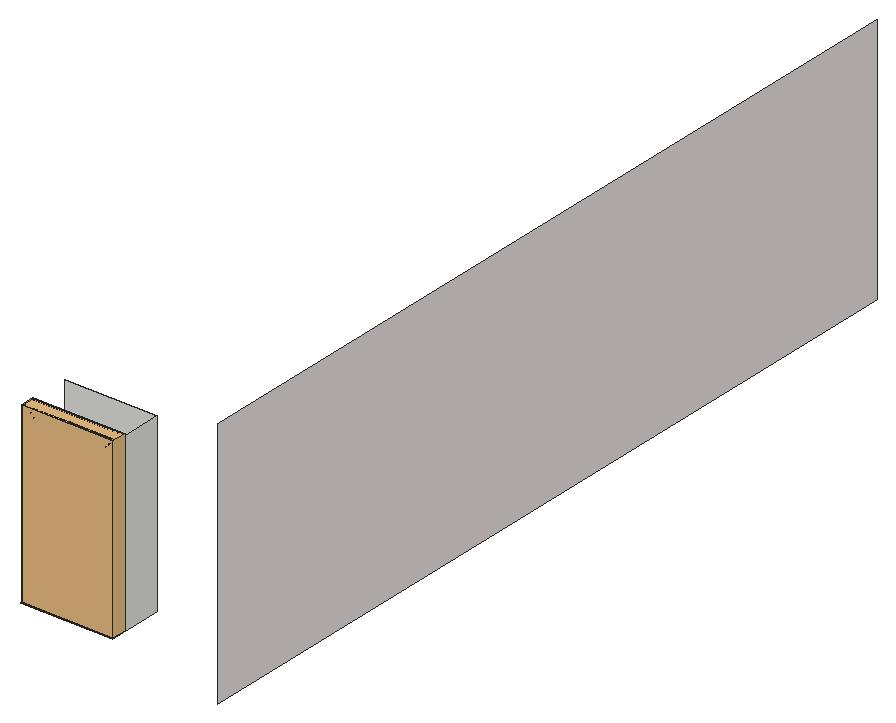
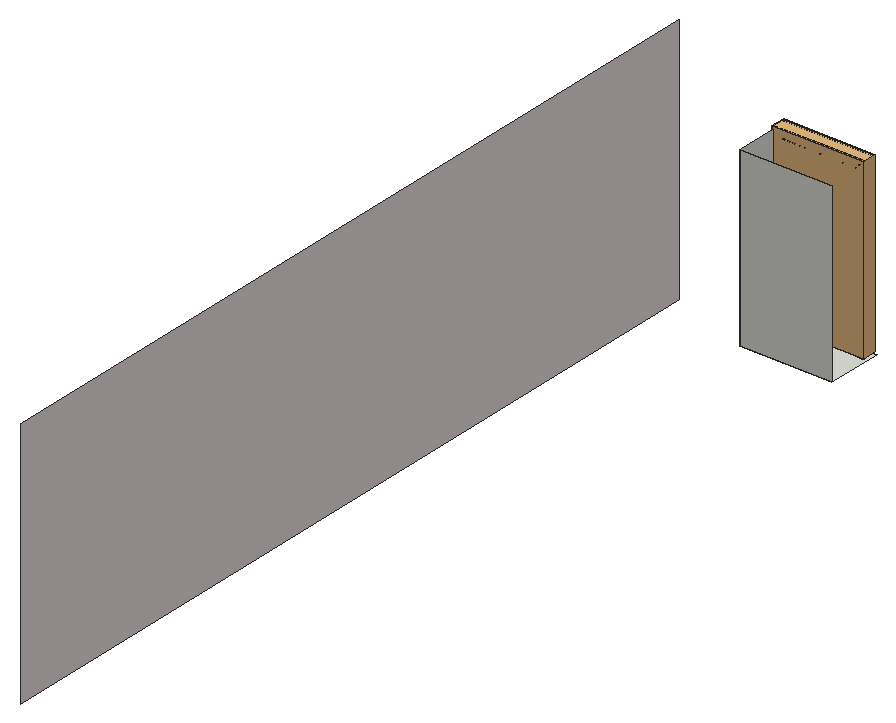
# SketchUp Ruby script. Lengths in inches.
U = 1.inch
M = Sketchup.active_model
def pt(a) = Geom::Point3d.new(a.map { |v| v * U })
def face(e, loops, mat)
  f = e.add_face(loops[0].map { |a| pt(a) })
  loops[1..].each { |l| e.add_face(l.map { |a| pt(a) }).erase! }
  f.material = f.back_material = mat if mat
  f
end
# faces: each face lists its corners as indices into pts; further lists are holes
def faces(e, pts, list, mat = nil) = list.each { |f| face(e, (f[0].is_a?(Array) ? f : [f]).map { |l| l.map { |i| pts[i] } }, mat) }
# xy, xz, yz: faces in a plane at the given z, y or x. An outline is a flat list of corners, or four numbers for a rectangle; further outlines are holes
def ring(l) = l.size == 4 ? [[l[0], l[1]], [l[2], l[1]], [l[2], l[3]], [l[0], l[3]]] : l.each_slice(2).to_a
def flat(e, list, mat, &to3) = list.each { |f| face(e, (f[0].is_a?(Array) ? f : [f]).map { |l| ring(l).map { |u, v| to3.(u, v) } }, mat) }
def xy(e, z, list, mat = nil) = flat(e, list, mat) { |x, y| [x, y, z] }
def xz(e, y, list, mat = nil) = flat(e, list, mat) { |x, z| [x, y, z] }
def yz(e, x, list, mat = nil) = flat(e, list, mat) { |y, z| [x, y, z] }
def lines(e, pts, list) = list.each { |a, b| e.add_line(pt(pts[a]), pt(pts[b])) }
# prism: a flat outline (further loops are holes) pulled along v
def prism(e, loops, v, mat = nil)
  f = face(e, loops, mat); d = Geom::Vector3d.new(v.map { |x| x * U })
  f.pushpull(f.normal.samedirection?(d) ? d.length : -d.length)
end
def box(e, o, s, mat = nil) = prism(e, [[o, [o[0] + s[0], o[1], o[2]], [o[0] + s[0], o[1] + s[1], o[2]], [o[0], o[1] + s[1], o[2]]]], [0, 0, s[2]], mat)
def at(x, y, z, deg = 0) = Geom::Transformation.translation(pt([x, y, z])) * Geom::Transformation.rotation(ORIGIN, Z_AXIS, deg.degrees)
def axes(o, x, y, z) = Geom::Transformation.new([*x, 0, *y, 0, *z, 0, *pt(o).to_a, 1])
def part(name) = M.definitions.add(name)
# library, detail: a bought-in or finely detailed component or shape, given as its bounding box
def library(name, o, s) = part(name).tap { |d| box(d.entities, o, s) }
def detail(e, o, s) = box(e.add_group.entities, o, s)
def put(e, d, t, mat = nil) = e.add_instance(d, t).tap { |i| i.material = mat if mat }
def group(e, t, mat = nil) = e.add_group.tap { |g| g.transformation = t; g.material = mat if mat }.entities
root = M.entities
M.materials.add("Generic\#5").color = [232, 222, 222]
M.materials.add("Material \#0").color = [86, 53, 35]
M.materials.add("Material \#1").color = [140, 140, 140]
c1 = part("3DGeom~19_Defintion")
xy(c1.entities,0,[[-6.28,-215.79,-994.45,-208.55,-13.52,-208.55],[-994.45,-215.79,-994.45,-208.55,-6.28,-215.79],[-6.28,-215.79,-13.52,-208.55,-13.52,0],[-6.28,-215.79,-13.52,0,-6.28,0],[-13.52,0,-13.52,208.55,-6.28,215.79],
  [-13.52,0,-6.28,215.79,-6.28,0],[-994.45,208.55,-6.28,215.79,-13.52,208.55],[-994.45,208.55,-994.45,215.79,-6.28,215.79]],"Material \#0")
p = [[-13.52,-208.55,0],[-994.45,-208.55,0],[-994.45,-207.81,0.07],[-14.25,-207.81,0.07],[-13.52,-208.55,0],[-14.25,-207.81,0.07],
  [-14.25,0,0.07],[-13.52,0,0],[-13.52,208.55,0],[-14.25,207.81,0.07],[-13.52,208.55,0],[-14.25,207.81,0.07],
  [-994.45,207.81,0.07],[-994.45,208.55,0],[-994.45,-207.21,0.27],[-994.45,-207.21,0.27],[-14.86,-207.21,0.27],[-14.86,-207.21,0.27],
  [-14.86,0,0.27],[-14.86,0,0.27],[-14.86,0,0.27],[-14.86,0,0.27],[-14.86,207.21,0.27],[-14.86,207.21,0.27],
  [-994.45,207.21,0.27],[-994.45,207.21,0.27],[-14.86,-207.21,0.27],[-994.45,-207.21,0.27],[-994.45,-206.74,0.6],[-15.33,-206.74,0.6],
  [-14.86,-207.21,0.27],[-15.33,-206.74,0.6],[-15.33,0,0.6],[-14.86,0,0.27],[-14.86,207.21,0.27],[-15.33,206.74,0.6],
  [-14.86,207.21,0.27],[-15.33,206.74,0.6],[-994.45,206.74,0.6],[-994.45,207.21,0.27],[-994.45,-206.4,1.07],[-15.66,-206.4,1.07],
  [-15.66,-206.4,1.07],[-15.66,0,1.07],[-15.66,206.4,1.07],[-15.66,206.4,1.07],[-994.45,206.4,1.07],[-994.45,-206.2,1.68],
  [-15.86,-206.2,1.68],[-15.86,-206.2,1.68],[-15.86,0,1.68],[-15.86,206.2,1.68],[-15.86,206.2,1.68],[-994.45,206.2,1.68],
  [-994.45,-206.13,2.41],[-15.93,-206.13,2.41],[-15.93,-206.13,2.41],[-15.93,0,2.41],[-15.93,206.13,2.41],[-15.93,206.13,2.41],
  [-994.45,206.13,2.41],[-994.45,-206.13,71.16],[-994.45,-206.22,71.59],[-15.79,-206.28,71.53],[-15.79,-206.28,71.53],[-15.84,0,71.59],
  [-15.93,0,71.16],[-15.79,206.28,71.53],[-15.79,206.28,71.53],[-994.45,206.22,71.59],[-994.45,206.13,71.16],[-15.79,-206.28,71.53],
  [-994.45,-206.48,71.84],[-994.45,-206.9,71.93],[-15.16,-206.9,71.93],[-15.79,-206.28,71.53],[-15.79,-206.28,71.53],[-15.16,-206.9,71.93],
  [-15.16,0,71.93],[-994.45,-206.48,71.84],[-15.59,0,71.84],[-15.79,-206.28,71.53],[-15.59,0,71.84],[-15.79,206.28,71.53],
  [-15.16,206.9,71.93],[-15.59,0,71.84],[-15.79,206.28,71.53],[-994.45,206.48,71.84],[-15.79,206.28,71.53],[-15.16,206.9,71.93],
  [-994.45,206.9,71.93],[-994.45,206.48,71.84],[-15.79,206.28,71.53],[-994.45,-227.27,72.01],[5.41,-227.47,72.33],[4.78,-226.84,71.93],
  [4.78,-226.84,71.93],[5.41,-227.47,72.33],[5.21,0,72.01],[-994.45,-226.84,71.93],[-994.45,-227.27,72.01],[5.21,0,72.01],
  [4.78,0,71.93],[4.78,226.84,71.93],[5.21,0,72.01],[5.21,0,72.01],[5.41,227.47,72.33],[4.78,226.84,71.93],
  [5.41,227.47,72.33],[-994.45,227.27,72.01],[-994.45,227.27,72.01],[-994.45,226.84,71.93],[-994.45,-227.27,72.01],[-994.45,-227.53,72.27],
  [5.41,-227.47,72.33],[5.41,-227.47,72.33],[5.47,0,72.27],[5.21,0,72.01],[5.41,227.47,72.33],[5.41,227.47,72.33],
  [-994.45,227.53,72.27],[-994.45,227.27,72.01],[-994.45,-227.61,72.7],[-994.45,-227.61,74.4375],[-994.45,-227.61,74.4375],[5.55,-227.61,74.4375],
  [5.55,-227.61,74.4375],[5.55,0,74.4375],[5.55,0,72.7],[5.55,227.61,74.4375],[5.55,227.61,74.4375],[-994.45,227.61,74.4375],
  [-994.45,227.61,74.4375],[-994.45,227.61,72.7]]
faces(c1.entities,p,[[0,1,2],[2,3,0],[4,5,6],[6,7,4],[8,7,6],[6,9,8],[10,11,12],[12,13,10],
  [3,2,14],[15,16,3],[5,17,18],[19,6,5],[9,6,20],[21,22,9],[11,23,24],[25,12,11],
  [26,27,28],[28,29,26],[30,31,32],[32,33,30],[34,33,32],[32,35,34],[36,37,38],[38,39,36],
  [29,28,40],[40,41,29],[31,42,43],[43,32,31],[35,32,43],[43,44,35],[37,45,46],[46,38,37],
  [41,40,47],[47,48,41],[42,49,50],[50,43,42],[44,43,50],[50,51,44],[45,52,53],[53,46,45],
  [48,47,54],[54,55,48],[49,56,57],[57,50,49],[51,50,57],[57,58,51],[52,59,60],[60,53,52],
  [61,62,63],[64,65,66],[66,65,67],[68,69,70],[71,72,73],[73,74,75],[76,77,78],[62,79,63],
  [78,80,76],[81,82,65],[83,80,78],[78,84,83],[65,85,86],[68,87,69],[88,89,90],[90,91,92],
  [93,94,95],[96,97,98],[95,99,100],[101,102,96],[103,102,104],[105,106,103],[107,108,109],[110,111,107],
  [112,113,114],[115,116,117],[117,116,118],[119,120,121],[114,122,123],[124,125,114],[113,122,114],[115,126,127],
  [127,128,115],[115,128,116],[118,128,127],[127,129,118],[116,128,118],[119,130,131],[132,133,119],[119,133,120]],"Material \#0")
c2 = part("3DGeom~15_Defintion")
xy(c2.entities,0,[[-961.58,-251.9,-958.5,-248.8125,-961.58,-237.8],[-961.58,-251.9,28.8,-248.8125,-958.5,-248.8125],[-961.58,-251.9,36.25,-251.9,28.8,-248.8125],[36.25,-251.9,19.98,-239.99,28.8,-248.8125],[36.25,-251.9,22.16,-237.8,19.98,-239.99],
  [-958.5,-248.8125,-958.5,-237.8,-961.58,-237.8],[19.98,-239.99,22.16,-237.8,3.36,-223.37],[-958.5,-237.8,-958.5,-223.37,-961.58,-220.28],[-961.58,-237.8,-958.5,-237.8,-961.58,-220.28],[22.16,-237.8,4.64,-220.28,3.36,-223.37],
  [-958.5,-223.37,4.64,-220.28,-961.58,-220.28],[-958.5,-223.37,3.36,-223.37,4.64,-220.28],[5.29,-219.63,8.375,-218.35,5.29,0],[8.375,-218.35,8.375,0,5.29,0],[5.29,0,8.375,0,5.29,219.63],
  [8.375,0,8.375,218.35,5.29,219.63],[8.375,218.35,22.8125,237.15,5.29,219.63],[-961.58,220.28,-958.5,223.37,-961.58,237.8],[-961.58,220.28,3.36,223.37,-958.5,223.37],[-961.58,220.28,4.64,220.28,3.36,223.37],
  [4.64,220.28,19.98,239.99,3.36,223.37],[4.64,220.28,22.16,237.8,19.98,239.99],[-958.5,223.37,-958.5,237.8,-961.58,237.8],[-958.5,237.8,-958.5,248.8125,-961.58,251.9],[-961.58,237.8,-958.5,237.8,-961.58,251.9],
  [22.16,237.8,28.8,248.8125,19.98,239.99],[22.16,237.8,36.25,251.9,28.8,248.8125],[-958.5,248.8125,36.25,251.9,-961.58,251.9],[-958.5,248.8125,28.8,248.8125,36.25,251.9]],"Material \#0")
xy(c2.entities,7.48,[[-962.79,-238.36,23.37,-238.36,-962.79,-219.67],[23.37,-238.36,4.67,-219.67,-962.79,-219.67],[23.37,-238.36,23.37,0,4.67,-219.67],[4.67,-219.67,23.37,0,4.67,0],[23.37,0,23.37,238.36,4.67,219.67],
  [4.67,0,23.37,0,4.67,219.67],[-962.79,219.67,23.37,238.36,-962.79,238.36],[-962.79,219.67,4.67,219.67,23.37,238.36]],"Material \#0")
xy(c2.entities,63.5625,[[-962.79,-238.36,-962.79,-219.67,4.67,-219.67],[-962.79,-238.36,4.67,-219.67,23.37,-238.36],[23.37,-238.36,4.67,-219.67,23.37,0],[4.67,-219.67,4.67,0,23.37,0],[23.37,0,4.67,219.67,23.37,238.36],
  [4.67,0,4.67,219.67,23.37,0],[-962.79,219.67,-962.79,238.36,4.67,219.67],[4.67,219.67,-962.79,238.36,23.37,238.36]],"Material \#0")
xy(c2.entities,69.64,[[-962.79,-219.62,4.63,-219.62,-962.79,-200.32],[4.63,-219.62,-14.68,-200.32,-962.79,-200.32],[4.63,-219.62,4.63,0,-14.68,-200.32],[-14.68,-200.32,4.63,0,-14.68,0],[-14.68,0,4.63,0,-14.68,200.32],
  [4.63,0,4.63,219.62,-14.68,200.32],[-962.79,200.32,-14.68,200.32,4.63,219.62],[-962.79,200.32,4.63,219.62,-962.79,219.62]],"Material \#0")
xy(c2.entities,71.04,[[-961.58,-251.9,-958.5,-248.8125,28.8,-248.8125],[-961.58,-251.9,-961.58,-237.8,-958.5,-248.8125],[-961.58,-251.9,28.8,-248.8125,36.25,-251.9],[36.25,-251.9,19.98,-239.99,22.16,-237.8],[36.25,-251.9,28.8,-248.8125,19.98,-239.99],
  [-958.5,-248.8125,-961.58,-237.8,-958.5,-237.8],[19.98,-239.99,3.36,-223.37,22.16,-237.8],[-958.5,-237.8,-961.58,-220.28,-958.5,-223.37],[-961.58,-237.8,-961.58,-220.28,-958.5,-237.8],[22.16,-237.8,3.36,-223.37,4.64,-220.28],
  [-958.5,-223.37,-961.58,-220.28,4.64,-220.28],[-958.5,-223.37,4.64,-220.28,3.36,-223.37],[5.29,-219.63,5.29,0,8.375,-218.35],[8.375,-218.35,5.29,0,8.375,0],[5.29,0,5.29,219.63,8.375,0],
  [8.375,0,5.29,219.63,8.375,218.35],[8.375,218.35,5.29,219.63,22.8125,237.15],[-961.58,220.28,-958.5,223.37,3.36,223.37],[-961.58,220.28,-961.58,237.8,-958.5,223.37],[-961.58,220.28,3.36,223.37,4.64,220.28],
  [4.64,220.28,3.36,223.37,19.98,239.99],[4.64,220.28,19.98,239.99,22.16,237.8],[-958.5,223.37,-961.58,237.8,-958.5,237.8],[-958.5,237.8,-961.58,251.9,-958.5,248.8125],[-961.58,237.8,-961.58,251.9,-958.5,237.8],
  [22.16,237.8,19.98,239.99,28.8,248.8125],[22.16,237.8,28.8,248.8125,36.25,251.9],[-958.5,248.8125,-961.58,251.9,36.25,251.9],[-958.5,248.8125,36.25,251.9,28.8,248.8125]],"Material \#0")
xz(c2.entities,-238.36,[[-962.79,63.5625,23.37,63.5625,23.37,72.07],[-962.79,63.5625,23.37,72.07,-962.79,72.07]],"Material \#0")
xz(c2.entities,-219.67,[[-962.79,7.48,4.67,7.48,-962.79,63.5625],[4.67,7.48,4.67,63.5625,-962.79,63.5625]],"Material \#0")
xz(c2.entities,219.67,[[-962.79,7.48,-962.79,63.5625,4.67,7.48],[4.67,7.48,-962.79,63.5625,4.67,63.5625]],"Material \#0")
xz(c2.entities,238.36,[[-962.79,63.5625,-962.79,72.07,23.37,72.07],[-962.79,63.5625,23.37,72.07,23.37,63.5625]],"Material \#0")
yz(c2.entities,4.67,[[-219.67,7.48,0,7.48,-219.67,63.5625],[0,7.48,0,63.5625,-219.67,63.5625],[0,7.48,219.67,63.5625,0,63.5625],[0,7.48,219.67,7.48,219.67,63.5625]],"Material \#0")
yz(c2.entities,23.37,[[-238.36,63.5625,0,63.5625,-238.36,72.07],[0,63.5625,0,72.07,-238.36,72.07],[0,63.5625,238.36,63.5625,238.36,72.07],[0,63.5625,238.36,72.07,0,72.07]],"Material \#0")
p = [[36.9,-251.24,0],[37.21,0,-0.16],[34.125,0,-0.14],[36.9,251.24,0],[33.83,243.81,0.02],[33.83,-243.8,0.02],
  [22.8125,-237.15,0],[24.99,-234.97,-0.01],[5.375,-220.37,0],[23.37,-238.36,7.48],[4.67,-219.67,7.48],[4.67,-219.67,7.48],
  [23.37,-238.36,7.48],[23.37,-238.36,0],[4.67,-219.67,7.48],[23.37,-238.36,0],[5.375,-220.37,0],[5.375,-220.37,0],
  [23.37,-238.36,0],[5.29,-219.63,0],[8.375,-218.35,0],[-15.36,-199.64,1.62],[4.67,-219.67,7.48],[5.375,-220.37,0],
  [-13.8,-201.19,0.06],[5.375,-220.37,0],[5.375,-220.37,0],[-14.84,-200.15,0.58],[5.375,-220.37,0],[-13.8,-201.19,0.06],
  [-6.08,-208.92,0],[5.375,-220.37,0],[-13.8,-201.19,0.06],[-6.08,-208.92,0],[-13.8,-201.19,0.06],[5.375,-220.37,0],
  [-6.08,-208.92,0],[-13.8,-201.19,0.06],[-13.09,-201.91,0],[-6.08,-208.92,0],[-13.09,-201.91,0],[-13.8,-201.19,0.06],
  [-15.36,199.64,1.62],[4.67,219.67,7.48],[5.375,220.37,0],[-13.8,201.19,0.06],[5.375,220.37,0],[5.375,220.37,0],
  [4.67,219.67,7.48],[-14.84,200.15,0.58],[5.375,220.37,0],[-13.8,201.19,0.06],[-6.08,208.92,0],[-13.09,201.91,0],
  [-13.8,201.19,0.06],[-6.08,208.92,0],[-13.8,201.19,0.06],[5.375,220.37,0],[-6.08,208.92,0],[5.375,220.37,0],
  [-13.8,201.19,0.06],[-6.08,208.92,0],[-13.8,201.19,0.06],[-13.09,201.91,0],[8.375,218.35,0],[24.99,234.97,-0.01],
  [22.8125,237.15,0],[23.37,238.36,7.48],[23.37,238.36,0],[23.37,238.36,0],[5.375,220.37,0],[5.375,220.37,0],
  [23.37,238.36,7.48],[4.67,219.67,7.48],[5.375,220.37,0],[23.37,238.36,0],[23.37,238.36,7.48],[-13.8,-201.19,0.06],
  [-14.84,-200.15,0.58],[-14.38,-200.61,0.26],[-13.8,-201.19,0.06],[-13.8,-201.19,0.06],[-14.38,-200.61,0.26],[-13.8,201.19,0.06],
  [-14.84,200.15,0.58],[-13.8,201.19,0.06],[-14.38,200.61,0.26],[-14.38,200.61,0.26],[-13.8,201.19,0.06],[4.63,-219.62,69.64],
  [4.63,-219.62,69.64],[-15.42,-199.57,9.43],[-15.36,-199.64,1.62],[-15.16,-199.83,1.04],[-15.16,-199.83,1.04],[-15.16,199.83,1.04],
  [-15.36,199.64,1.62],[-15.16,199.83,1.04],[-15.42,199.57,9.43],[4.63,219.62,69.64],[4.67,219.67,7.48],[4.63,219.62,69.64],
  [4.63,-219.62,69.64],[4.67,-219.67,63.5625],[4.67,-219.67,63.5625],[4.67,-219.67,7.48],[-15.28,-199.71,69.25],[4.63,-219.62,69.64],
  [-15.42,-199.57,9.43],[-15.28,-199.71,69.25],[-15.42,-199.57,2.34],[-15.42,-199.57,2.34],[-15.42,199.57,2.34],[-15.42,199.57,9.43],
  [-15.28,199.71,69.25],[-15.28,199.71,69.25],[4.63,219.62,69.64],[4.63,219.62,69.64],[4.67,219.67,63.5625],[4.67,219.67,63.5625],
  [-15.42,199.57,2.34],[4.67,-219.67,63.5625],[4.63,-219.62,69.64],[4.67,219.67,7.48],[4.67,219.67,63.5625],[4.63,219.62,69.64],
  [4.63,-219.62,69.64],[-15.28,-199.71,69.25],[-15.28,-199.71,69.25],[-15.42,-199.57,48.99],[-15.42,-199.57,48.99],[-15.28,-199.71,69.25],
  [-15.42,199.57,48.99],[-15.28,199.71,69.25],[-15.28,199.71,69.25],[-15.42,199.57,48.99],[4.63,219.62,69.64],[4.63,-219.62,69.64],
  [23.37,-238.36,72.07],[4.67,-219.67,63.5625],[4.67,-219.67,63.5625],[23.37,-238.36,63.5625],[23.37,-238.36,72.07],[4.67,-219.67,63.5625],
  [5.24,-220.23,70.03],[23.37,-238.36,72.07],[23.37,-238.36,63.5625],[4.67,-219.67,63.5625],[4.67,-219.67,63.5625],[4.63,-219.62,69.64],
  [4.63,219.62,69.64],[23.37,238.36,72.07],[4.67,219.67,63.5625],[4.67,219.67,63.5625],[5.24,220.23,70.03],[4.63,219.62,69.64],
  [23.37,238.36,63.5625],[4.67,219.67,63.5625],[4.67,219.67,63.5625],[23.37,238.36,63.5625],[23.37,238.36,72.07],[4.67,219.67,63.5625],
  [23.37,238.36,72.07],[4.63,-219.62,69.64],[-14.68,-200.32,69.64],[-15.28,-199.71,69.25],[-15.28,-199.71,69.25],[-14.68,-200.32,69.64],
  [4.63,-219.62,69.64],[-15.28,199.71,69.25],[-14.68,200.32,69.64],[4.63,219.62,69.64],[4.63,219.62,69.64],[-14.68,200.32,69.64],
  [4.63,-219.62,69.64],[5.24,-220.23,70.03],[23.37,-238.36,72.07],[4.63,219.62,69.64],[5.24,220.23,70.03],[5.375,-220.37,72.07],
  [5.375,-220.37,72.07],[23.37,-238.36,72.07],[5.375,220.37,72.07],[23.37,238.36,72.07],[5.375,220.37,72.07],[33.83,-243.8,71.03],
  [36.9,-251.24,71.04],[22.8125,-237.15,71.04],[34.125,0,71.19],[37.21,0,71.2],[24.99,-234.97,71.05],[5.29,-219.63,71.04],
  [8.375,-218.35,71.04],[33.83,243.81,71.03],[36.9,251.24,71.04],[22.8125,237.15,71.04],[24.99,234.97,71.05],[8.375,218.35,71.04]]
faces(c2.entities,p,[[0,1,2],[1,3,4],[4,2,1],[2,5,0],[6,0,5],[5,7,6],[8,9,10],[11,12,13],
  [14,15,16],[17,18,9],[19,6,7],[7,20,19],[21,22,23],[24,21,25],[26,10,27],[28,27,29],
  [30,31,32],[33,34,35],[36,37,38],[39,40,41],[42,43,44],[45,42,46],[47,48,49],[50,49,51],
  [52,53,54],[55,56,57],[58,59,60],[61,62,63],[64,65,66],[43,67,68],[43,69,70],[71,72,73],
  [74,75,76],[3,66,65],[65,4,3],[77,78,21],[27,79,80],[81,82,78],[83,84,42],[85,86,84],
  [49,87,88],[10,89,27],[90,91,27],[92,93,27],[91,92,27],[78,94,21],[84,95,42],[96,97,49],
  [98,96,49],[99,98,49],[100,101,49],[21,102,103],[21,104,105],[21,106,107],[21,108,109],[91,110,92],
  [21,111,108],[42,112,113],[42,113,114],[42,115,116],[42,117,118],[42,119,43],[98,120,96],[10,121,122],
  [123,124,125],[126,127,91],[128,129,91],[108,130,131],[113,132,133],[134,135,98],[136,134,98],[137,138,139],
  [140,141,142],[143,142,144],[145,146,147],[148,144,149],[150,151,152],[153,154,155],[151,156,157],[158,159,160],
  [161,162,154],[163,164,165],[166,167,168],[169,170,171],[172,173,134],[174,175,176],[177,178,151],[142,179,144],
  [175,180,181],[178,182,151],[183,184,154],[185,186,187],[186,185,188],[188,189,186],[187,190,185],[190,187,191],
  [191,192,190],[189,188,193],[193,194,189],[195,196,197],[196,195,194],[194,193,196]],"Material \#0")
c3 = part("3DGeom~22_Defintion")
xz(c3.entities,-210.625,[[-1016.13,2.47,-1016.13,9.96,-16.28,2.47],[-16.28,2.47,-1016.13,9.96,-16.28,9.96],[-1016.13,9.96,-1016.13,51.7,-16.28,51.7],[-1016.13,9.96,-16.28,51.7,-16.28,9.96],[-1016.13,51.7,-1016.13,72.71,-16.28,51.7]],"Material \#0")
xz(c3.entities,210.625,[[-1016.13,2.47,-16.28,2.47,-1016.13,9.96],[-16.28,2.47,-16.28,9.96,-1016.13,9.96],[-1016.13,9.96,-16.28,51.7,-1016.13,51.7],[-1016.13,9.96,-16.28,9.96,-16.28,51.7],[-1016.13,51.7,-16.28,51.7,-1016.13,72.71]],"Material \#0")
yz(c3.entities,-16.28,[[-210.625,2.47,-210.625,9.96,0,9.96],[-210.625,2.47,0,9.96,0,2.47],[0,2.47,0,9.96,210.625,2.47],[210.625,2.47,0,9.96,210.625,9.96],[-210.625,9.96,-210.625,51.7,0,51.7],
  [-210.625,9.96,0,51.7,0,9.96],[0,9.96,0,51.7,210.625,9.96],[210.625,9.96,0,51.7,210.625,51.7],[-210.625,51.7,0,72.71,0,51.7],[0,51.7,0,72.71,210.625,51.7]],"Material \#0")
p = [[-1016.13,-210.625,72.71],[-16.13,-210.77,73.09],[-16.28,-210.625,51.7],[-16.28,-210.625,51.7],[-16.13,-210.77,73.09],[-16.28,0,72.71],
  [-16.13,210.77,73.09],[-16.28,210.625,51.7],[-16.28,210.625,51.7],[-16.13,210.77,73.09],[-1016.13,210.625,72.71]]
faces(c3.entities,p,[[0,1,2],[3,4,5],[5,6,7],[8,9,10]],"Material \#0")
c4 = library("3DGeom~16_Defintion",[-962.62,-252.34,-11.22],[1000,504.68,93.46])
c5 = part("3DGeom~17_Defintion")
yz(c5.entities,-1908.8,[[-436.03,-21.87,-436.73,-21.5,-435.91,-21.83],[436.03,-21.87,435.91,-21.83,436.73,-21.5],[-435.91,-21.83,-436.73,-21.5,-436.15,-21.125],[-435.91,-21.83,-436.15,-21.125,-435.87,-21.72],[435.91,-21.83,435.87,-21.72,436.15,-21.125],
  [435.91,-21.83,436.15,-21.125,436.73,-21.5],[-436.73,-21.5,-484.73,-21.37,-436.15,-1.11],[-471.46,-21.5,-484.73,-21.37,-436.73,-21.5],[-477.2,-21.5,-484.73,-21.37,-471.46,-21.5],[-481.82,-21.5,-484.73,-21.37,-477.2,-21.5],
  [-436.73,-21.5,-436.15,-1.11,-436.15,-21.125],[436.73,-21.5,436.15,-21.125,471.46,-21.5],[471.46,-21.5,436.15,-21.125,477.2,-21.5],[477.2,-21.5,436.15,-21.125,499.98,-0.85],[477.2,-21.5,499.98,-0.85,481.82,-21.5],
  [481.82,-21.5,487.35,-21,484.73,-21.37],[481.82,-21.5,491.8,-19.52,487.35,-21],[481.82,-21.5,497.64,-13.67,491.8,-19.52],[481.82,-21.5,499.98,-0.85,497.64,-13.67],[-484.73,-21.37,-498.5,-11.58,-499.84,-0.37],
  [-484.73,-21.37,-499.84,-0.37,-499.4,-0.5],[-484.73,-21.37,-499.4,-0.5,-436.15,-1.11],[-484.73,-21.37,-493.63,-18.42,-498.5,-11.58],[-484.73,-21.37,-489.71,-20.375,-493.63,-18.42],[-484.73,-21.37,-487.35,-21,-489.71,-20.375],
  [436.15,-21.125,436.15,-1.11,436.73,-0.74],[436.15,-21.125,436.73,-0.74,499.98,-0.85],[487.35,-21,491.8,-19.52,489.71,-20.375],[-489.71,-20.375,-491.8,-19.52,-493.63,-18.42],[491.8,-19.52,495.21,-17.08,493.63,-18.42],
  [491.8,-19.52,497.64,-13.67,495.21,-17.08],[-493.63,-18.42,-496.54,-15.5,-498.5,-11.58],[-493.63,-18.42,-495.21,-17.08,-496.54,-15.5],[495.21,-17.08,497.64,-13.67,496.54,-15.5],[-496.54,-15.5,-497.64,-13.67,-498.5,-11.58],
  [497.64,-13.67,499.125,-9.22,498.5,-11.58],[497.64,-13.67,499.625,-3.69,499.125,-9.22],[497.64,-13.67,499.98,-0.85,499.625,-3.69],[-498.5,-11.58,-499.625,-3.69,-499.84,-0.37],[-498.5,-11.58,-499.5,-6.6,-499.625,-3.69],
  [-498.5,-11.58,-499.125,-9.22,-499.5,-6.6],[499.125,-9.22,499.625,-3.69,499.5,-6.6],[-499.625,-3.69,-499.98,-0.85,-500,-0.52],[-499.625,-3.69,-500,-0.52,-499.84,-0.37],[-436.15,-1.11,-499.4,-0.5,-471.46,-0.74],
  [-436.15,-1.11,-471.46,-0.74,-436.73,-0.74],[-436.15,-1.11,-436.73,-0.74,-435.91,-0.41],[-436.15,-1.11,-435.91,-0.41,-435.87,-0.52],[436.15,-1.11,435.87,-0.52,435.91,-0.41],[436.15,-1.11,435.91,-0.41,436.73,-0.74],
  [499.98,-0.85,436.73,-0.74,471.46,-0.74],[499.98,-0.85,471.46,-0.74,499.4,-0.5],[499.98,-0.85,499.4,-0.5,499.96,-0.41],[499.98,-0.85,499.96,-0.41,500,-0.52],[-436.73,-0.74,-436.03,-0.37,-435.91,-0.41],
  [436.73,-0.74,435.91,-0.41,436.03,-0.37],[-500,-0.52,-499.96,-0.41,-499.84,-0.37],[499.4,-0.5,499.84,-0.37,499.96,-0.41],[-499.84,141.21,-499.96,141.25,-499.4,141.35],[-436.03,141.21,-436.73,141.59,-435.91,141.25],
  [436.03,141.21,435.91,141.25,436.73,141.59],[499.84,141.21,484.73,162.21,498.5,152.42],[499.84,141.21,499.4,141.35,484.73,162.21],[499.84,141.21,498.5,152.42,499.625,144.53],[499.84,141.21,499.625,144.53,500,141.37],
  [499.84,141.21,500,141.37,499.96,141.25],[-499.96,141.25,-500,141.37,-499.98,141.69],[-499.96,141.25,-499.98,141.69,-499.4,141.35],[-435.91,141.25,-436.73,141.59,-436.15,141.96],[-435.91,141.25,-436.15,141.96,-435.87,141.37],
  [435.91,141.25,435.87,141.37,436.15,141.96],[435.91,141.25,436.15,141.96,436.73,141.59],[-499.4,141.35,-499.98,141.69,-471.46,141.59],[499.4,141.35,436.15,141.96,484.73,162.21],[499.4,141.35,471.46,141.59,436.15,141.96],
  [500,141.37,499.625,144.53,499.98,141.69],[-436.73,141.59,-499.98,141.69,-436.15,161.97],[-471.46,141.59,-499.98,141.69,-436.73,141.59],[-436.73,141.59,-436.15,161.97,-436.15,141.96],[436.73,141.59,436.15,141.96,471.46,141.59],
  [-499.98,141.69,-477.2,162.34,-436.15,161.97],[-499.98,141.69,-481.82,162.34,-477.2,162.34],[-499.98,141.69,-497.64,154.51,-481.82,162.34],[-499.98,141.69,-499.625,144.53,-497.64,154.51],[436.15,141.96,436.15,161.97,436.73,162.34],
  [436.15,141.96,436.73,162.34,484.73,162.21],[-499.625,144.53,-499.125,150.07,-497.64,154.51],[-499.625,144.53,-499.5,147.44,-499.125,150.07],[499.625,144.53,498.5,152.42,499.5,147.44],[499.5,147.44,498.5,152.42,499.125,150.07],
  [-499.125,150.07,-498.5,152.42,-497.64,154.51],[498.5,152.42,484.73,162.21,493.63,159.26],[498.5,152.42,493.63,159.26,496.54,156.34],[498.5,152.42,496.54,156.34,497.64,154.51],[-497.64,154.51,-491.8,160.36,-481.82,162.34],
  [-497.64,154.51,-495.21,157.92,-491.8,160.36],[-497.64,154.51,-496.54,156.34,-495.21,157.92],[496.54,156.34,493.63,159.26,495.21,157.92],[-495.21,157.92,-493.63,159.26,-491.8,160.36],[493.63,159.26,484.73,162.21,489.71,161.22],
  [493.63,159.26,489.71,161.22,491.8,160.36],[-491.8,160.36,-487.35,161.84,-481.82,162.34],[-491.8,160.36,-489.71,161.22,-487.35,161.84],[489.71,161.22,484.73,162.21,487.35,161.84],[-487.35,161.84,-484.73,162.21,-481.82,162.34],
  [-436.15,161.97,-477.2,162.34,-471.46,162.34],[-436.15,161.97,-471.46,162.34,-436.73,162.34],[-436.15,161.97,-436.73,162.34,-435.91,162.68],[-436.15,161.97,-435.91,162.68,-435.87,162.56],[436.15,161.97,435.87,162.56,435.91,162.68],
  [436.15,161.97,435.91,162.68,436.73,162.34],[484.73,162.21,436.73,162.34,471.46,162.34],[484.73,162.21,471.46,162.34,477.2,162.34],[484.73,162.21,477.2,162.34,481.82,162.34],[-436.73,162.34,-436.03,162.72,-435.91,162.68],
  [436.73,162.34,435.91,162.68,436.03,162.72]],"Material \#0")
c6 = part("3DGeom~18_Defintion")
xz(c6.entities,-241.71,[[-976.3,0,23.7,0,23.7,7.58],[-976.3,0,23.7,7.58,-976.3,7.58]],"Material \#0")
xz(c6.entities,241.71,[[-976.3,0,-976.3,7.58,23.7,7.58],[-976.3,0,23.7,7.58,23.7,0]],"Material \#0")
yz(c6.entities,23.7,[[-241.71,0,0,0,-241.71,7.58],[0,0,0,7.58,-241.71,7.58],[0,0,241.71,0,241.71,7.58],[0,0,241.71,7.58,0,7.58]],"Material \#0")
c7 = part("3DGeom~20_Defintion")
xy(c7.entities,0,[[-976.3,-241.71,-976.3,-223.46,23.7,-241.71],[23.7,-241.71,-976.3,-223.46,5.45,-223.46],[23.7,-241.71,5.45,-223.46,5.45,0],[23.7,-241.71,5.45,0,23.7,0],[-976.3,-223.46,-976.3,-211.85,5.45,-223.46],
  [5.45,-223.46,-976.3,-211.85,-6.16,-211.85],[5.45,-223.46,-6.16,-211.85,-6.16,0],[5.45,-223.46,-6.16,0,5.45,0],[-6.16,0,-6.16,211.85,5.45,223.46],[-6.16,0,5.45,223.46,5.45,0],
  [5.45,0,23.7,241.71,23.7,0],[5.45,0,5.45,223.46,23.7,241.71],[-976.3,211.85,-976.3,223.46,5.45,223.46],[-976.3,211.85,5.45,223.46,-6.16,211.85],[-976.3,223.46,-976.3,241.71,23.7,241.71],
  [-976.3,223.46,23.7,241.71,5.45,223.46]],"Material \#0")
xy(root,151.7789,[[330.35,114.8125,374.475,141.3125]])
xz(root,116.631,[[338.0558,187.3364,338.1814,187.3593,338.0558,187.3483],[338.0558,187.3364,338.1836,187.3476,338.1814,187.3593],[338.1836,187.3476,338.2993,187.3908,338.1814,187.3593],[338.1836,187.3476,338.3036,187.3796,338.2993,187.3908],[338.3036,187.3796,338.408,187.441,338.2993,187.3908],
  [338.3036,187.3796,338.4142,187.4307,338.408,187.441],[338.4142,187.4307,338.5055,187.508,338.408,187.441],[338.4142,187.4307,338.5134,187.499,338.5055,187.508],[338.5134,187.499,338.5897,187.59,338.5055,187.508],[338.5134,187.499,338.5991,187.5823,338.5897,187.59],
  [338.0558,187.5212,338.0959,187.5366,338.0558,187.5331],[338.0558,187.5212,338.0981,187.5249,338.0959,187.5366],[338.0981,187.5249,338.1339,187.5468,338.0959,187.5366],[338.0981,187.5249,338.1381,187.5356,338.1339,187.5468],[338.1381,187.5356,338.1688,187.5629,338.1339,187.5468],
  [338.1381,187.5356,338.175,187.5526,338.1688,187.5629],[338.175,187.5526,338.2,187.5844,338.1688,187.5629],[338.175,187.5526,338.2079,187.5753,338.2,187.5844],[338.2079,187.5753,338.2269,187.6105,338.2,187.5844],[338.2079,187.5753,338.2363,187.6029,338.2269,187.6105],
  [338.2363,187.6029,338.249,187.6409,338.2269,187.6105],[338.2363,187.6029,338.2596,187.6349,338.249,187.6409],[338.2596,187.6349,338.2656,187.6749,338.249,187.6409],[338.2881,187.7097,338.2796,187.7507,338.2761,187.7118],[338.2881,187.7097,338.2919,187.7507,338.2796,187.7507],
  [338.2796,187.7507,338.2919,187.7507,338.2761,187.7897],[338.2656,187.8266,338.2771,187.8308,338.249,187.8606],[338.2771,187.8308,338.2596,187.8666,338.249,187.8606],[338.249,187.8606,338.2596,187.8666,338.2269,187.8909],[338.2596,187.8666,338.2363,187.8986,338.2269,187.8909],
  [338.2269,187.8909,338.2363,187.8986,338.2,187.9171],[338.2363,187.8986,338.2079,187.9262,338.2,187.9171],[338.2,187.9171,338.2079,187.9262,338.1688,187.9386],[338.2079,187.9262,338.175,187.9488,338.1688,187.9386],[338.1688,187.9386,338.175,187.9488,338.1339,187.9547],
  [338.175,187.9488,338.1381,187.9659,338.1339,187.9547],[338.1339,187.9547,338.1381,187.9659,338.0959,187.9649],[338.0959,187.9649,338.0981,187.9766,338.0558,187.9684],[338.0959,187.9649,338.1381,187.9659,338.0981,187.9766],[338.0558,187.9684,338.0981,187.9766,338.0558,187.9803]],"Material \#1")
xz(root,116.6656,[[338.0558,189.7138,338.0912,189.7177,338.1237,189.729],[338.0558,189.7138,338.1237,189.729,338.1763,189.77],[338.1237,189.729,338.1523,189.7468,338.1763,189.77],[338.1763,189.77,338.0558,190.1601,338,190.1664],[338.1763,189.77,338.2102,189.8639,338.0558,190.1601],
  [338.1763,189.77,338.1945,189.7979,338.2061,189.8295],[338.1763,189.77,338.2061,189.8295,338.2102,189.8639],[338.2102,189.8639,338.1117,190.1664,338.0558,190.1601],[338.2102,189.8639,338.163,190.1842,338.1117,190.1664],[338.2102,189.8639,338.2082,190.2122,338.163,190.1842],
  [338.2102,189.8639,338.2102,190.151,338.2082,190.2122],[338.2102,190.151,338.2118,190.1636,338.2082,190.2122],[338.2102,190.151,338.2106,190.1576,338.2118,190.1636],[338.2118,190.1636,338.246,190.2489,338.2082,190.2122],[338.2118,190.1636,338.2137,190.1692,338.2165,190.1744],
  [338.2118,190.1636,338.2165,190.1744,338.246,190.2489],[338.2165,190.1744,338.2199,190.1792,338.3295,190.3617],[338.2165,190.1744,338.2748,190.2929,338.246,190.2489],[338.2165,190.1744,338.3295,190.3617,338.2748,190.2929],[338.2199,190.1792,338.2241,190.1839,338.3295,190.3617],
  [338.2241,190.1839,338.229,190.1883,338.2761,190.2374],[338.2241,190.1839,338.2761,190.2374,338.3295,190.3617],[338.229,190.1883,338.2539,190.2116,338.2761,190.2374],[338.2761,190.2374,338.2952,190.2655,338.3107,190.2957],[338.2761,190.2374,338.3107,190.2957,338.3295,190.3617],
  [338.2748,190.2929,338.3295,190.3617,338.2931,190.3428],[338.3107,190.2957,338.3223,190.3278,338.3295,190.3617],[338.2931,190.3428,338.3295,190.3617,338.2995,190.3971],[338.3295,190.3617,338.2713,190.565,338.2748,190.5012],[338.3295,190.3617,338.3247,190.4586,338.2713,190.565],
  [338.3295,190.3617,338.2748,190.5012,338.2931,190.4514],[338.3295,190.3617,338.2931,190.4514,338.2995,190.3971],[338.3295,190.3617,338.332,190.3971,338.3247,190.4586],[338.3247,190.4586,338.3039,190.5151,338.2713,190.565],[338.2748,190.5012,338.2713,190.565,338.246,190.5453],
  [338.246,190.5453,338.2713,190.565,338.2082,190.582],[338.2713,190.565,338.0558,190.6657,338.163,190.61],[338.2713,190.565,338.1772,190.6383,338.0558,190.6657],[338.2713,190.565,338.163,190.61,338.2082,190.582],[338.2713,190.565,338.2285,190.6066,338.1772,190.6383],
  [338.163,190.61,338.0558,190.6657,338.1117,190.6278],[338.1117,190.6278,338.0558,190.6657,338.0558,190.6341],[338.1772,190.6383,338.1191,190.6586,338.0558,190.6657]],"Material \#1")
xz(root,141.3125,[[330.35,151.7789,374.475,235.7164]])
yz(root,374.475,[[114.8125,151.7789,141.3125,235.7164]])
yz(root,424.8848,[[114.8125,141.9375,508.6875,261.9375]],"Generic\#5")
put(root,c1,axes([353.08,120.67,233.84],[0,0,0.08182],[0.08414,0,0],[0,-0.07149,0]),"Material \#0")
put(root,c2,axes([353.08,120.67,233.84],[0,0,0.08451],[0.0869,0,0],[0,-0.07384,0]),"Material \#0")
put(root,c3,axes([353.08,120.67,233.84],[0,0,0.08007],[0.08234,0,0],[0,-0.06996,0]),"Material \#0")
put(root,c4,axes([353.08,120.67,233.84],[0,0,0.08452],[0.08692,0,0],[0,-0.07385,0]),"Material \#0")
put(root,c5,axes([353.08,120.67,233.84],[0,0,0.04263],[0.04383,0,0],[0,-0.03724,0]),"Material \#0")
put(root,c6,axes([353.08,120.67,233.84],[0,0,0.08334],[0.0857,0,0],[0,-0.07281,0]),"Material \#0")
put(root,c7,axes([353.08,120.67,233.84],[0,0,0.08334],[0.0857,0,0],[0,-0.07281,0]),"Material \#0")
